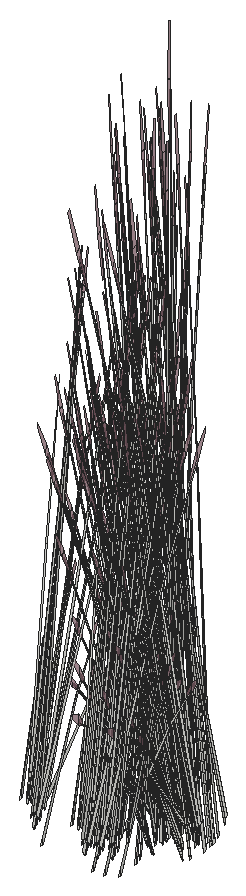
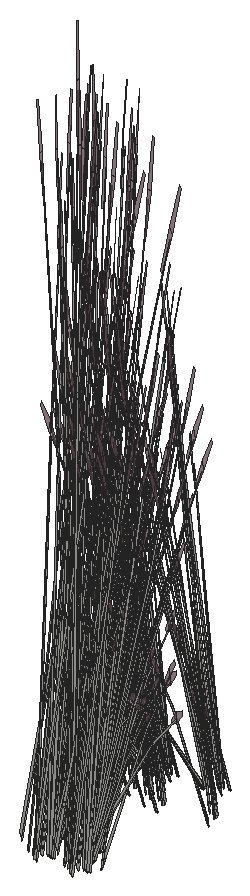
# SketchUp Ruby script. Lengths in inches.
U = 1.inch
M = Sketchup.active_model
def pt(a) = Geom::Point3d.new(a.map { |v| v * U })
def face(e, loops, mat)
  f = e.add_face(loops[0].map { |a| pt(a) })
  loops[1..].each { |l| e.add_face(l.map { |a| pt(a) }).erase! }
  f.material = f.back_material = mat if mat
  f
end
# faces: each face lists its corners as indices into pts; further lists are holes
def faces(e, pts, list, mat = nil) = list.each { |f| face(e, (f[0].is_a?(Array) ? f : [f]).map { |l| l.map { |i| pts[i] } }, mat) }
# xy, xz, yz: faces in a plane at the given z, y or x. An outline is a flat list of corners, or four numbers for a rectangle; further outlines are holes
def ring(l) = l.size == 4 ? [[l[0], l[1]], [l[2], l[1]], [l[2], l[3]], [l[0], l[3]]] : l.each_slice(2).to_a
def flat(e, list, mat, &to3) = list.each { |f| face(e, (f[0].is_a?(Array) ? f : [f]).map { |l| ring(l).map { |u, v| to3.(u, v) } }, mat) }
def xy(e, z, list, mat = nil) = flat(e, list, mat) { |x, y| [x, y, z] }
def xz(e, y, list, mat = nil) = flat(e, list, mat) { |x, z| [x, y, z] }
def yz(e, x, list, mat = nil) = flat(e, list, mat) { |y, z| [x, y, z] }
def lines(e, pts, list) = list.each { |a, b| e.add_line(pt(pts[a]), pt(pts[b])) }
# prism: a flat outline (further loops are holes) pulled along v
def prism(e, loops, v, mat = nil)
  f = face(e, loops, mat); d = Geom::Vector3d.new(v.map { |x| x * U })
  f.pushpull(f.normal.samedirection?(d) ? d.length : -d.length)
end
def box(e, o, s, mat = nil) = prism(e, [[o, [o[0] + s[0], o[1], o[2]], [o[0] + s[0], o[1] + s[1], o[2]], [o[0], o[1] + s[1], o[2]]]], [0, 0, s[2]], mat)
def at(x, y, z, deg = 0) = Geom::Transformation.translation(pt([x, y, z])) * Geom::Transformation.rotation(ORIGIN, Z_AXIS, deg.degrees)
def axes(o, x, y, z) = Geom::Transformation.new([*x, 0, *y, 0, *z, 0, *pt(o).to_a, 1])
def part(name) = M.definitions.add(name)
# library, detail: a bought-in or finely detailed component or shape, given as its bounding box
def library(name, o, s) = part(name).tap { |d| box(d.entities, o, s) }
def detail(e, o, s) = box(e.add_group.entities, o, s)
def put(e, d, t, mat = nil) = e.add_instance(d, t).tap { |i| i.material = mat if mat }
def group(e, t, mat = nil) = e.add_group.tap { |g| g.transformation = t; g.material = mat if mat }.entities
root = M.entities
M.materials.add("LightPink_Translucent").color = [144, 107, 117]
M.materials["LightPink_Translucent"].alpha = 0.75
c1 = part("blade")
p = [[2.15,0.21,22],[0,0.17,0],[0.09,0.45,0],[2.18,0.31,22],[2.29,0.31,22],[0.38,0.45,0],
  [2.48,0.24,33],[2.49,0.24,33],[2.48,0.22,33]]
faces(c1.entities,p,[[0,1,2,3],[4,5,2,3],[6,3,4,7],[8,0,3,6]])
c2 = part("seeds")
p = [[0.3,-0.1,1.38],[-0.01,-0.03,1.59],[-0.01,-0.03,0.03],[0.14,-0.07,-0.07],[0.29,-0.03,3],[0.15,0.01,3.11]]
faces(c2.entities,p,[[0,1,2,3],[1,0,4,5]],"LightPink_Translucent")
c3 = part("blade with seeds")
put(c3.entities,c1,at(0,0,0))
put(c3.entities,c2,axes([2.4,0.25,30.99],[1.5799,-0.05474,1.17369],[-0.12525,1.92788,0.29478],[-0.07173,-0.02425,1.56792]))
put(root,c3,axes([333.97,652.92,624.4375],[-0.00877,0.09229,1.74944],[0.24897,0.32105,-0.27667],[-0.06518,0.15182,0.14031]))
put(root,c3,axes([334.68,653.7,622.31],[0.11138,-0.07357,1.43002],[0.27499,0.22183,-0.30754],[-0.08185,0.19194,0.61141]))
put(root,c3,axes([334.79,652.99,624.25],[-0.23881,0.24554,-0.35414],[-0.22606,-0.28036,0.4572],[-0.0344,0.14245,0.87481]))
put(root,c3,axes([333.94,653.86,624.43],[0.04004,-0.02816,1.77383],[0.33095,0.18728,-0.16761],[-0.00778,0.15594,0.31391]))
put(root,c3,axes([334.95,652.73,625.0625],[-0.00918,0.43138,-0.7886],[-0.38672,-0.02897,0.09517],[-0.04081,0.18275,1.11556]))
put(root,c3,axes([334.95,653.94,622.49],[-0.00913,-0.2773,1.1486],[0.22824,0.19778,0.84392],[-0.04489,0.13217,0.25299]))
put(root,c3,axes([334.82,653.34,623.09],[0.00775,-0.24075,1.54345],[0.34877,0.12716,0.21329],[-0.03022,0.25658,0.72882]))
put(root,c3,axes([335.03,652.875,624.73],[0.25266,0.31335,-0.5672],[-0.2669,0.27442,-0.43934],[-0.03844,0.15921,1.08528]))
put(root,c3,axes([334.77,652.71,625.12],[0.3879,0.02311,-0.13498],[-0.0106,0.43749,-0.74919],[-0.02694,0.1685,1.13838]))
put(root,c3,axes([334.76,653.34,622.55],[0.32063,-0.08258,0.06507],[0.07371,0.33271,-0.86304],[-0.02033,0.16842,0.7736]))
put(root,c3,axes([335.32,652.42,623.6],[-0.00864,-0.17899,1.71376],[0.37441,0.11874,0.13857],[-0.02316,0.25508,0.73262]))
put(root,c3,axes([335.59,653.34,624.79],[-0.34777,-0.12192,0.53283],[0.11892,-0.40083,0.43934],[0.0209,0.15763,1.10256]))
put(root,c3,axes([339.11,661.4375,621.875],[0.14639,-0.01056,1.71376],[-0.09712,0.45778,0.13857],[-0.20862,-0.02831,0.73262]))
put(root,c3,axes([335.49,653.37,624.45],[-0.26007,0.1585,0.0643],[-0.12729,-0.28902,0.50621],[0.02512,0.1274,0.77189]))
put(root,c3,axes([335.55,653.28,621.22],[0.05712,-0.02538,1.76342],[0.34359,0.13968,-0.26939],[0.01005,0.15742,0.30037]))
put(root,c3,axes([335.625,653.42,624.25],[-0.1064,0.35863,-0.35414],[-0.31043,-0.1046,0.4572],[0.02846,0.14439,0.87481]))
put(root,c3,axes([335.4,654.06,624.4375],[0.04474,0.0751,1.74944],[0.36104,0.0295,-0.27667],[0.03631,0.16562,0.14031]))
put(root,c3,axes([339.55,661.01,622.98],[-0.35281,-0.01123,-0.71045],[0.0237,-0.47284,0.08574],[-0.14947,-0.0499,1.00501]))
put(root,c3,axes([339.26,661.125,620.59],[0.06891,0.12984,1.43002],[-0.15879,0.35293,-0.30754],[-0.16304,-0.08436,0.61141]))
put(root,c3,axes([339.39,660.7,621.875],[0.1311,0.08035,1.71376],[-0.27131,0.33708,0.13857],[-0.16909,-0.15206,0.73262]))
put(root,c3,axes([335.66,653.1,624.71],[0.16845,0.3792,-0.71045],[-0.34676,0.21133,0.08574],[0.03939,0.18322,1.00501]))
put(root,c3,axes([339.43,661.11,622.68],[-0.25628,0.30892,-0.51099],[-0.22444,-0.32634,-0.3958],[-0.13021,-0.047,0.97773]))
put(root,c3,axes([339.07,660.24,622.71],[0.02617,0.04654,1.77383],[-0.12614,0.41836,-0.16761],[-0.12775,0.00303,0.31391]))
put(root,c3,axes([335.78,653.18,624.4],[0.34695,0.11691,-0.51099],[-0.11892,0.40083,-0.3958],[0.03181,0.16138,0.97773]))
put(root,c3,axes([335.49,653.2,624.76],[0.34538,-0.21713,-0.1216],[0.16972,0.38536,-0.67495],[0.04557,0.16239,1.02557]))
put(root,c3,axes([339.36,659.96,622.72],[-0.07594,-0.00329,1.74944],[-0.24177,0.32918,-0.27667],[-0.129,-0.06726,0.14031]))
put(root,c3,axes([339.57,660.78,623.03],[-0.0189,0.47427,-0.1216],[-0.35781,-0.01296,-0.67495],[-0.13781,-0.03295,1.02557]))
put(root,c3,axes([339.34,660.82,622.53],[-0.20082,-0.29199,-0.35414],[0.2293,-0.2764,0.4572],[-0.1165,-0.04206,0.87481]))
put(root,c3,axes([338.85,661.52,620.77],[0.22533,-0.03337,1.1486],[-0.14293,0.29403,0.84392],[-0.11135,-0.04411,0.25299]))
put(root,c3,axes([338.43,652.92,623.9375],[-0.00877,0.09229,1.74944],[0.24897,0.32105,-0.27667],[-0.06518,0.15182,0.14031]))
put(root,c3,axes([339.31,660.71,623.09],[0.29147,-0.34417,0.53763],[0.25138,0.3655,0.4433],[-0.13675,-0.06349,1.11249]))
put(root,c3,axes([335.98,652.35,623.6],[-0.08068,-0.14973,1.71376],[0.3728,-0.12606,0.13857],[0.08426,0.23506,0.73262]))
put(root,c3,axes([339.4375,660.71,622.73],[0.01777,-0.35463,0.0643],[0.26836,0.00972,0.50621],[-0.1028,-0.03711,0.77189]))
put(root,c3,axes([340.2,662.66,620.06],[-0.36714,-0.07646,-0.62353],[0.07747,-0.47163,-0.16365],[-0.10956,-0.05715,1.37633]))
put(root,c3,axes([340.26,660.09,623.43],[-0.23555,0.44708,-0.13619],[-0.34112,-0.25757,-0.75594],[-0.11858,-0.12631,1.14864]))
put(root,c3,axes([339.62,660.97,623.05],[0.20082,0.29199,0.35414],[-0.2293,0.2764,-0.4572],[-0.1165,-0.04206,0.87481]))
put(root,c3,axes([340.16,660.45,622.98],[-0.30095,-0.22541,-0.71045],[0.21388,-0.395,0.08574],[-0.10904,-0.13459,1.00501]))
put(root,c3,axes([340.02,660.47,622.68],[-0.34827,0.11086,-0.51099],[-0.06092,-0.41983,-0.3958],[-0.09354,-0.12031,0.97773]))
put(root,c3,axes([339.14,653.7,621.81],[0.11138,-0.07357,1.43002],[0.27499,0.22183,-0.30754],[-0.08185,0.19194,0.61141]))
put(root,c3,axes([339.57,660.08,619.49],[-0.03419,0.06144,1.76342],[-0.3455,0.13246,-0.26939],[-0.08346,-0.12049,0.30037]))
put(root,c3,axes([339.26,652.99,623.75],[-0.23881,0.24554,-0.35414],[-0.22606,-0.28036,0.4572],[-0.0344,0.14245,0.87481]))
put(root,c3,axes([339.36,660.32,620.13],[-0.10181,0.3808,-0.03893],[-0.31336,-0.11714,-0.17649],[-0.04758,-0.06228,0.58215]))
put(root,c3,axes([340.17,659.03,622.71],[-0.00658,0.0559,1.77383],[-0.32474,0.20287,-0.16761],[-0.09556,-0.1037,0.31391]))
put(root,c3,axes([339.51,652.92,624.03],[-0.00877,0.09229,1.74944],[0.24897,0.32105,-0.27667],[-0.06518,0.15182,0.14031]))
put(root,c3,axes([338.4,653.86,623.93],[0.04004,-0.02816,1.77383],[0.33095,0.18728,-0.16761],[-0.00778,0.15594,0.31391]))
put(root,c3,axes([339.82,659.84,620.59],[-0.02137,0.15256,1.43002],[-0.31245,0.12771,-0.30754],[-0.07303,-0.19719,0.61141]))
put(root,c3,axes([339.93,660.24,621.875],[0.08068,0.14973,1.71376],[-0.3728,0.12606,0.13857],[-0.08426,-0.23506,0.73262]))
put(root,c3,axes([340.06,660.16,622.53],[-0.05451,-0.37564,-0.35414],[0.31161,-0.09919,0.4572],[-0.0837,-0.10765,0.87481]))
put(root,c3,axes([339.1875,662.06,620.375],[-0.44133,0,0],[0,-0.52122,-0.51607],[0,-0.11871,1.63711]))
put(root,c3,axes([339.41,652.73,624.5625],[-0.00918,0.43138,-0.7886],[-0.38672,-0.02897,0.09517],[-0.04081,0.18275,1.11556]))
put(root,c3,axes([339.41,653.94,621.99],[-0.00913,-0.2773,1.1486],[0.22824,0.19778,0.84392],[-0.04489,0.13217,0.25299]))
put(root,c3,axes([342.22,661.42,621.875],[0.14639,-0.01056,1.71376],[-0.09712,0.45778,0.13857],[-0.20862,-0.02831,0.73262]))
put(root,c3,axes([340.24,660.46,623.05],[0.05451,0.37564,0.35414],[-0.31161,0.09919,-0.4572],[-0.0837,-0.10765,0.87481]))
put(root,c3,axes([339.53,661.92,620.33],[-0.32829,0.39208,0.30756],[-0.32849,-0.38796,-0.36492],[-0.01146,-0.11134,1.64885]))
put(root,c3,axes([339.28,653.34,622.59],[0.00775,-0.24075,1.54345],[0.34877,0.12716,0.21329],[-0.03022,0.25658,0.72882]))
put(root,c3,axes([340.88,663,621.33],[0.305,0.18805,1.51261],[-0.29879,0.40513,0.59816],[-0.13384,-0.24012,1.26806]))
put(root,c3,axes([339.72,659.59,620.77],[0.18411,0.16231,1.1486],[-0.26813,0.09757,0.84392],[-0.05737,-0.12474,0.25299]))
put(root,c3,axes([340.39,662.51,620.21],[-0.21202,-0.39143,-0.44739],[0.32115,-0.27564,0.21531],[-0.06861,-0.04843,1.43643]))
put(root,c3,axes([340.22,653.7,621.91],[0.11138,-0.07357,1.43002],[0.27499,0.22183,-0.30754],[-0.08185,0.19194,0.61141]))
put(root,c3,axes([340.1,660.02,623.09],[0.39316,-0.11987,0.53763],[0.06823,0.47021,0.4433],[-0.09247,-0.13858,1.11249]))
put(root,c3,axes([339.49,652.875,624.23],[0.25266,0.31335,-0.5672],[-0.2669,0.27442,-0.43934],[-0.03844,0.15921,1.08528]))
put(root,c3,axes([340.19,660.12,622.73],[0.16041,-0.29625,0.0643],[0.22843,0.17248,0.50621],[-0.07385,-0.09498,0.77189]))
put(root,c3,axes([340.42,662.74,620.4375],[0.09355,-0.55261,-0.23429],[0.44354,0.09633,0.51271],[-0.0775,-0.07631,1.5644]))
put(root,c3,axes([339.23,652.71,624.62],[0.3879,0.02311,-0.13498],[-0.0106,0.43749,-0.74919],[-0.02694,0.1685,1.13838]))
put(root,c3,axes([340.33,652.99,623.84],[-0.23881,0.24554,-0.35414],[-0.22606,-0.28036,0.4572],[-0.0344,0.14245,0.87481]))
put(root,c3,axes([339.22,653.34,622.05],[0.32063,-0.08258,0.06507],[0.07371,0.33271,-0.86304],[-0.02033,0.16842,0.7736]))
put(root,c3,axes([340.54,659.24,622.72],[-0.05398,-0.06539,1.74944],[-0.36026,0.04145,-0.27667],[-0.0575,-0.15639,0.14031]))
put(root,c3,axes([339.29,661.7,620.02],[0,-0.46636,-0.49651],[0.39487,0,0],[0,-0.10622,1.57504]))
put(root,c3,axes([339.46,662.14,620.48],[0,0.46636,0.49651],[-0.39487,0,0],[0,-0.10622,1.57504]))
put(root,c3,axes([339.78,652.42,623.1],[-0.00864,-0.17899,1.71376],[0.37441,0.11874,0.13857],[-0.02316,0.25508,0.73262]))
put(root,c3,axes([342.66,660.99,622.98],[-0.35281,-0.01123,-0.71045],[0.0237,-0.47284,0.08574],[-0.14947,-0.0499,1.00501]))
put(root,c3,axes([339.48,653.86,624.03],[0.04004,-0.02816,1.77383],[0.33095,0.18728,-0.16761],[-0.00778,0.15594,0.31391]))
put(root,c3,axes([342.38,661.11,620.59],[0.06891,0.12984,1.43002],[-0.15879,0.35293,-0.30754],[-0.16304,-0.08436,0.61141]))
put(root,c3,axes([340.32,662.24,620.67],[-0.39748,-0.22252,-0.29095],[0.19139,-0.46966,-0.50002],[-0.01249,-0.11531,1.59708]))
put(root,c3,axes([342.5,660.68,621.875],[0.1311,0.08035,1.71376],[-0.27131,0.33708,0.13857],[-0.16909,-0.15206,0.73262]))
put(root,c3,axes([340.49,652.73,624.66],[-0.00918,0.43138,-0.7886],[-0.38672,-0.02897,0.09517],[-0.04081,0.18275,1.11556]))
put(root,c3,axes([340.84,652.92,624.42],[-0.00877,0.09229,1.74944],[0.24897,0.32105,-0.27667],[-0.06518,0.15182,0.14031]))
put(root,c3,axes([340.49,653.94,622.08],[-0.00913,-0.2773,1.1486],[0.22824,0.19778,0.84392],[-0.04489,0.13217,0.25299]))
put(root,c3,axes([340.14,661.77,620.1],[-0.14494,-0.47823,-0.69835],[0.41752,-0.17223,-0.18329],[-0.01602,-0.16194,1.54149]))
put(root,c3,axes([341.09,660.25,623.03],[-0.34538,0.21713,-0.1216],[-0.16972,-0.38536,-0.67495],[-0.04557,-0.16239,1.02557]))
put(root,c3,axes([340.79,660.27,622.68],[-0.34695,-0.11691,-0.51099],[0.11892,-0.40083,-0.3958],[-0.03181,-0.16138,0.97773]))
put(root,c3,axes([342.55,661.09,622.68],[-0.25628,0.30892,-0.51099],[-0.22444,-0.32634,-0.3958],[-0.13021,-0.047,0.97773]))
put(root,c3,axes([339.46,661.71,620.03],[0.24637,-0.29097,-0.30978],[0.24637,0.29097,0.30978],[0,-0.09372,1.38974]))
put(root,c3,axes([342.18,660.22,622.71],[0.02617,0.04654,1.77383],[-0.12614,0.41836,-0.16761],[-0.12775,0.00303,0.31391]))
put(root,c3,axes([340.57,659.83,620.13],[-0.2439,0.26754,-0.03893],[-0.22348,-0.29302,-0.17649],[-0.01573,-0.08303,0.58215]))
put(root,c3,axes([340.36,653.34,622.68],[0.00775,-0.24075,1.54345],[0.34877,0.12716,0.21329],[-0.03022,0.25658,0.72882]))
put(root,c3,axes([340.05,653.34,624.29],[-0.34777,-0.12192,0.53283],[0.11892,-0.40083,0.43934],[0.0209,0.15763,1.10256]))
put(root,c3,axes([342.48,659.94,622.72],[-0.07594,-0.00329,1.74944],[-0.24177,0.32918,-0.27667],[-0.129,-0.06726,0.14031]))
put(root,c3,axes([339.95,653.37,623.95],[-0.26007,0.1585,0.0643],[-0.12729,-0.28902,0.50621],[0.02512,0.1274,0.77189]))
put(root,c3,axes([340.36,662.37,620.72],[-0.17124,0.42022,0.44739],[-0.35581,-0.20224,-0.21531],[0,-0.09687,1.43643]))
put(root,c3,axes([340.92,660.35,622.98],[-0.16845,-0.3792,-0.71045],[0.34676,-0.21133,0.08574],[-0.03939,-0.18322,1.00501]))
put(root,c3,axes([342.68,660.76,623.03],[-0.0189,0.47427,-0.1216],[-0.35781,-0.01296,-0.67495],[-0.13781,-0.03295,1.02557]))
put(root,c3,axes([342.45,660.8,622.53],[-0.20082,-0.29199,-0.35414],[0.2293,-0.2764,0.4572],[-0.1165,-0.04206,0.87481]))
put(root,c3,axes([340.57,652.875,624.32],[0.25266,0.31335,-0.5672],[-0.2669,0.27442,-0.43934],[-0.03844,0.15921,1.08528]))
put(root,c3,axes([341.97,661.5,620.77],[0.22533,-0.03337,1.1486],[-0.14293,0.29403,0.84392],[-0.11135,-0.04411,0.25299]))
put(root,c3,axes([340.99,660.4,623.05],[-0.1064,0.35863,0.35414],[-0.31043,-0.1046,-0.4572],[-0.02846,-0.14439,0.87481]))
put(root,c3,axes([341.55,653.7,622.3],[0.11138,-0.07357,1.43002],[0.27499,0.22183,-0.30754],[-0.08185,0.19194,0.61141]))
put(root,c3,axes([340.01,653.28,620.72],[0.05712,-0.02538,1.76342],[0.34359,0.13968,-0.26939],[0.01005,0.15742,0.30037]))
put(root,c3,axes([340.31,652.71,624.71],[0.3879,0.02311,-0.13498],[-0.0106,0.43749,-0.74919],[-0.02694,0.1685,1.13838]))
put(root,c3,axes([340.08,653.42,623.75],[-0.1064,0.35863,-0.35414],[-0.31043,-0.1046,0.4572],[0.02846,0.14439,0.87481]))
put(root,c3,axes([340.3,653.34,622.14],[0.32063,-0.08258,0.06507],[0.07371,0.33271,-0.86304],[-0.02033,0.16842,0.7736]))
put(root,c3,axes([342.42,660.6875,623.09],[0.29147,-0.34417,0.53763],[0.25138,0.3655,0.4433],[-0.13675,-0.06349,1.11249]))
put(root,c3,axes([340.86,652.42,623.19],[-0.00864,-0.17899,1.71376],[0.37441,0.11874,0.13857],[-0.02316,0.25508,0.73262]))
put(root,c3,axes([340.63,659.51,619.49],[-0.0592,0.0168,1.76342],[-0.32738,-0.18913,-0.26939],[0.00549,-0.15776,0.30037]))
put(root,c3,axes([341.67,652.99,624.23],[-0.23881,0.24554,-0.35414],[-0.22606,-0.28036,0.4572],[-0.0344,0.14245,0.87481]))
put(root,c3,axes([340.95,660.02,622.53],[0.1064,-0.35863,-0.35414],[0.31043,0.1046,0.4572],[-0.02846,-0.14439,0.87481]))
put(root,c3,axes([340.43,661.96,620.36],[0.15345,0.52148,0.45755],[-0.43845,0.18134,0.17955],[0.00536,-0.09582,1.58856]))
put(root,c3,axes([339.86,654.06,623.9375],[0.04474,0.0751,1.74944],[0.36104,0.0295,-0.27667],[0.03631,0.16562,0.14031]))
put(root,c3,axes([340.36,661.89,620.21],[0.17124,-0.42022,-0.44739],[0.35581,0.20224,0.21531],[0,-0.09687,1.43643]))
put(root,c3,axes([342.55,660.68,622.73],[0.01777,-0.35463,0.0643],[0.26836,0.00972,0.50621],[-0.1028,-0.03711,0.77189]))
put(root,c3,axes([340.82,653.86,624.42],[0.04004,-0.02816,1.77383],[0.33095,0.18728,-0.16761],[-0.00778,0.15594,0.31391]))
put(root,c3,axes([343.3125,662.64,620.06],[-0.36714,-0.07646,-0.62353],[0.07747,-0.47163,-0.16365],[-0.10956,-0.05715,1.37633]))
put(root,c3,axes([343.38,660.07,623.43],[-0.23555,0.44708,-0.13619],[-0.34112,-0.25757,-0.75594],[-0.11858,-0.12631,1.14864]))
put(root,c3,axes([342.74,660.95,623.05],[0.20082,0.29199,0.35414],[-0.2293,0.2764,-0.4572],[-0.1165,-0.04206,0.87481]))
put(root,c3,axes([343.28,660.43,622.98],[-0.30095,-0.22541,-0.71045],[0.21388,-0.395,0.08574],[-0.10904,-0.13459,1.00501]))
put(root,c3,axes([343.14,660.44,622.68],[-0.34827,0.11086,-0.51099],[-0.06092,-0.41983,-0.3958],[-0.09354,-0.12031,0.97773]))
put(root,c3,axes([341.83,652.73,625.05],[-0.00918,0.43138,-0.7886],[-0.38672,-0.02897,0.09517],[-0.04081,0.18275,1.11556]))
put(root,c3,axes([340.12,653.1,624.21],[0.16845,0.3792,-0.71045],[-0.34676,0.21133,0.08574],[0.03939,0.18322,1.00501]))
put(root,c3,axes([341.125,653.34,624.38],[-0.34777,-0.12192,0.53283],[0.11892,-0.40083,0.43934],[0.0209,0.15763,1.10256]))
put(root,c3,axes([341.08,660.08,622.73],[0.26007,-0.1585,0.0643],[0.12729,0.28902,0.50621],[-0.02512,-0.1274,0.77189]))
put(root,c3,axes([341.82,653.94,622.47],[-0.00913,-0.2773,1.1486],[0.22824,0.19778,0.84392],[-0.04489,0.13217,0.25299]))
put(root,c3,axes([342.6875,660.0625,619.49],[-0.03419,0.06144,1.76342],[-0.3455,0.13246,-0.26939],[-0.08346,-0.12049,0.30037]))
put(root,c3,axes([340.98,662.01,620.21],[0,-0.53961,0],[0.44133,0,0],[0,0,1.79456]))
put(root,c3,axes([341.03,653.37,624.05],[-0.26007,0.1585,0.0643],[-0.12729,-0.28902,0.50621],[0.02512,0.1274,0.77189]))
put(root,c3,axes([340.99,660.11,622.73],[0.34777,0.12192,0.48003],[-0.11892,0.40083,0.3958],[-0.0209,-0.15763,0.9933]))
put(root,c3,axes([340.57,662.1,620.43],[0.39767,0.22603,0.24065],[-0.19139,0.46966,0.50002],[0,-0.10827,1.60543]))
put(root,c3,axes([340.45,661.79,620.72],[-0.38326,0.02879,0.44739],[-0.03466,-0.47788,-0.21531],[0.06861,-0.04843,1.43643]))
put(root,c3,axes([341.7,653.34,623.07],[0.00775,-0.24075,1.54345],[0.34877,0.12716,0.21329],[-0.03022,0.25658,0.72882]))
put(root,c3,axes([340.24,653.18,623.9],[0.34695,0.11691,-0.51099],[-0.11892,0.40083,-0.3958],[0.03181,0.16138,0.97773]))
put(root,c3,axes([339.95,653.2,624.26],[0.34538,-0.21713,-0.1216],[0.16972,0.38536,-0.67495],[0.04557,0.16239,1.02557]))
put(root,c3,axes([340.08,660.4,620.375],[-0.22066,-0.46731,0],[0.36918,-0.26061,-0.51607],[0.08408,-0.05936,1.63711]))
put(root,c3,axes([342.47,660.3,620.13],[-0.10181,0.3808,-0.03893],[-0.31336,-0.11714,-0.17649],[-0.04758,-0.06228,0.58215]))
put(root,c3,axes([341.09,653.28,620.81],[0.05712,-0.02538,1.76342],[0.34359,0.13968,-0.26939],[0.01005,0.15742,0.30037]))
put(root,c3,axes([341.16,653.42,623.84],[-0.1064,0.35863,-0.35414],[-0.31043,-0.1046,0.4572],[0.02846,0.14439,0.87481]))
put(root,c3,axes([343.29,659.01,622.71],[-0.00658,0.0559,1.77383],[-0.32474,0.20287,-0.16761],[-0.09556,-0.1037,0.31391]))
put(root,c3,axes([341.01,659.27,620.77],[0.04528,0.27194,1.1486],[-0.25117,-0.15062,0.84392],[0.02703,-0.13924,0.25299]))
put(root,c3,axes([341.91,652.875,624.71],[0.25266,0.31335,-0.5672],[-0.2669,0.27442,-0.43934],[-0.03844,0.15921,1.08528]))
put(root,c3,axes([342.9375,659.82,620.59],[-0.02137,0.15256,1.43002],[-0.31245,0.12771,-0.30754],[-0.07303,-0.19719,0.61141]))
put(root,c3,axes([343.04,660.21,621.875],[0.08068,0.14973,1.71376],[-0.3728,0.12606,0.13857],[-0.08426,-0.23506,0.73262]))
put(root,c3,axes([340.78,661.67,620.36],[-0.29264,0.42323,0.45755],[-0.34767,-0.3736,0.17955],[0.07055,-0.04224,1.58856]))
put(root,c3,axes([342.78,652.92,624.44],[-0.00877,0.09229,1.74944],[0.24897,0.32105,-0.27667],[-0.06518,0.15182,0.14031]))
put(root,c3,axes([343.17,660.14,622.53],[-0.05451,-0.37564,-0.35414],[0.31161,-0.09919,0.4572],[-0.0837,-0.10765,0.87481]))
put(root,c3,axes([342.3,662.04,620.375],[-0.44133,0,0],[0,-0.52122,-0.51607],[0,-0.11871,1.63711]))
put(root,c3,axes([341.64,652.71,625.1],[0.3879,0.02311,-0.13498],[-0.0106,0.43749,-0.74919],[-0.02694,0.1685,1.13838]))
put(root,c3,axes([342.08,659.71,622.71],[-0.03584,0.03562,1.77383],[-0.35118,-0.12018,-0.16761],[-0.01271,-0.15545,0.31391]))
put(root,c3,axes([340.94,654.06,624.03],[0.04474,0.0751,1.74944],[0.36104,0.0295,-0.27667],[0.03631,0.16562,0.14031]))
put(root,c3,axes([341.81,660.74,623.03],[-0.3879,-0.02311,-0.1216],[0.0106,-0.43749,-0.67495],[0.02694,-0.1685,1.02557]))
put(root,c3,axes([341.63,653.34,622.53],[0.32063,-0.08258,0.06507],[0.07371,0.33271,-0.86304],[-0.02033,0.16842,0.7736]))
put(root,c3,axes([342.19,652.42,623.58],[-0.00864,-0.17899,1.71376],[0.37441,0.11874,0.13857],[-0.02316,0.25508,0.73262]))
put(root,c3,axes([343.36,660.44,623.05],[0.05451,0.37564,0.35414],[-0.31161,0.09919,-0.4572],[-0.0837,-0.10765,0.87481]))
put(root,c3,axes([341.66,660.81,623.05],[-0.23881,0.24554,0.35414],[-0.22606,-0.28036,-0.4572],[0.0344,-0.14245,0.87481]))
put(root,c3,axes([342.64,661.9,620.33],[-0.32829,0.39208,0.30756],[-0.32849,-0.38796,-0.36492],[-0.01146,-0.11134,1.64885]))
put(root,c3,axes([340.52,661.6875,620.67],[-0.04113,-0.53214,-0.29095],[0.42835,-0.03218,-0.50002],[0.07543,-0.07088,1.59708]))
put(root,c3,axes([340.4375,652.35,623.1],[-0.08068,-0.14973,1.71376],[0.3728,-0.12606,0.13857],[0.08426,0.23506,0.73262]))
put(root,c3,axes([341.54,660.57,622.68],[-0.25266,-0.31335,-0.51099],[0.2669,-0.27442,-0.3958],[0.03844,-0.15921,0.97773]))
put(root,c3,axes([344,662.98,621.33],[0.305,0.18805,1.51261],[-0.29879,0.40513,0.59816],[-0.13384,-0.24012,1.26806]))
put(root,c3,axes([342.83,659.57,620.77],[0.18411,0.16231,1.1486],[-0.26813,0.09757,0.84392],[-0.05737,-0.12474,0.25299]))
put(root,c3,axes([343.5,662.49,620.21],[-0.21202,-0.39143,-0.44739],[0.32115,-0.27564,0.21531],[-0.06861,-0.04843,1.43643]))
put(root,c3,axes([341.19,653.1,624.3],[0.16845,0.3792,-0.71045],[-0.34676,0.21133,0.08574],[0.03939,0.18322,1.00501]))
put(root,c3,axes([340.46,660.51,620.03],[0.32928,0.11539,-0.30978],[-0.08291,0.40636,0.30978],[0.06638,-0.04686,1.38974]))
put(root,c3,axes([343.22,660,623.09],[0.39316,-0.11987,0.53763],[0.06823,0.47021,0.4433],[-0.09247,-0.13858,1.11249]))
put(root,c3,axes([341.38,660.02,620.59],[-0.10032,0.0944,1.43002],[-0.30046,-0.16522,-0.30754],[0.05569,-0.20547,0.61141]))
put(root,c3,axes([343.49,653.7,622.32],[0.11138,-0.07357,1.43002],[0.27499,0.22183,-0.30754],[-0.08185,0.19194,0.61141]))
put(root,c3,axes([343.31,660.1,622.73],[0.16041,-0.29625,0.0643],[0.22843,0.17248,0.50621],[-0.07385,-0.09498,0.77189]))
put(root,c3,axes([340.38,660.32,620.02],[0.33032,-0.23318,-0.49651],[0.19744,0.41812,0],[0.07523,-0.05311,1.57504]))
put(root,c3,axes([343.53,662.72,620.4375],[0.09355,-0.55261,-0.23429],[0.44354,0.09633,0.51271],[-0.0775,-0.07631,1.5644]))
put(root,c3,axes([342.46,653.34,624.77],[-0.34777,-0.12192,0.53283],[0.11892,-0.40083,0.43934],[0.0209,0.15763,1.10256]))
put(root,c3,axes([341.32,653.18,624],[0.34695,0.11691,-0.51099],[-0.11892,0.40083,-0.3958],[0.03181,0.16138,0.97773]))
put(root,c3,axes([341.02,653.2,624.35],[0.34538,-0.21713,-0.1216],[0.16972,0.38536,-0.67495],[0.04557,0.16239,1.02557]))
put(root,c3,axes([342.37,653.37,624.4375],[-0.26007,0.1585,0.0643],[-0.12729,-0.28902,0.50621],[0.02512,0.1274,0.77189]))
put(root,c3,axes([341.52,660.76,620.48],[-0.33032,-0.23318,0.49651],[0.19744,-0.41812,0],[0.07523,0.05311,1.57504]))
put(root,c3,axes([341.62,660.72,622.98],[0.00918,-0.43138,-0.71045],[0.38672,0.02897,0.08574],[0.04081,-0.18275,1.00501]))
put(root,c3,axes([343.66,659.22,622.72],[-0.05398,-0.06539,1.74944],[-0.36026,0.04145,-0.27667],[-0.0575,-0.15639,0.14031]))
put(root,c3,axes([342.4,661.68,620.02],[0,-0.46636,-0.49651],[0.39487,0,0],[0,-0.10622,1.57504]))
put(root,c3,axes([342.57,662.12,620.48],[0,0.46636,0.49651],[-0.39487,0,0],[0,-0.10622,1.57504]))
put(root,c3,axes([343.6,652.99,624.25],[-0.23881,0.24554,-0.35414],[-0.22606,-0.28036,0.4572],[-0.0344,0.14245,0.87481]))
put(root,c3,axes([343.43,662.22,620.67],[-0.39748,-0.22252,-0.29095],[0.19139,-0.46966,-0.50002],[-0.01249,-0.11531,1.59708]))
put(root,c3,axes([342.75,653.86,624.43],[0.04004,-0.02816,1.77383],[0.33095,0.18728,-0.16761],[-0.00778,0.15594,0.31391]))
put(root,c3,axes([342.42,653.28,621.2],[0.05712,-0.02538,1.76342],[0.34359,0.13968,-0.26939],[0.01005,0.15742,0.30037]))
put(root,c3,axes([342.5,653.42,624.23],[-0.1064,0.35863,-0.35414],[-0.31043,-0.1046,0.4572],[0.02846,0.14439,0.87481]))
put(root,c3,axes([341.78,660.46,622.53],[0.23881,-0.24554,-0.35414],[0.22606,0.28036,0.4572],[0.0344,-0.14245,0.87481]))
put(root,c3,axes([341.87,660.58,622.73],[0.29004,0.02173,0.0643],[-0.00795,0.32812,0.50621],[0.03035,-0.12569,0.77189]))
put(root,c3,axes([343.26,661.75,620.1],[-0.14494,-0.47823,-0.69835],[0.41752,-0.17223,-0.18329],[-0.01602,-0.16194,1.54149]))
put(root,c3,axes([344.21,660.23,623.03],[-0.34538,0.21713,-0.1216],[-0.16972,-0.38536,-0.67495],[-0.04557,-0.16239,1.02557]))
put(root,c3,axes([343.91,660.25,622.68],[-0.34695,-0.11691,-0.51099],[0.11892,-0.40083,-0.3958],[-0.03181,-0.16138,0.97773]))
put(root,c3,axes([342.16,660.04,622.72],[-0.00341,-0.09282,1.74944],[-0.28775,-0.26825,-0.27667],[0.04449,-0.16261,0.14031]))
put(root,c3,axes([340.78,661.28,620.06],[0.23773,-0.35053,-0.62353],[0.29532,0.31785,-0.16365],[0.09526,-0.08744,1.37633]))
put(root,c3,axes([341.78,660.55,622.73],[0.25132,0.3182,0.48003],[-0.2669,0.27442,0.3958],[0.04636,-0.14929,0.9933]))
put(root,c3,axes([343.76,652.73,625.0625],[-0.00918,0.43138,-0.7886],[-0.38672,-0.02897,0.09517],[-0.04081,0.18275,1.11556]))
put(root,c3,axes([343.75,653.94,622.49],[-0.00913,-0.2773,1.1486],[0.22824,0.19778,0.84392],[-0.04489,0.13217,0.25299]))
put(root,c3,axes([342.57,661.69,620.03],[0.24637,-0.29097,-0.30978],[0.24637,0.29097,0.30978],[0,-0.09372,1.38974]))
put(root,c3,axes([343.68,659.8125,620.13],[-0.2439,0.26754,-0.03893],[-0.22348,-0.29302,-0.17649],[-0.01573,-0.08303,0.58215]))
put(root,c3,axes([341.52,652.35,623.19],[-0.08068,-0.14973,1.71376],[0.3728,-0.12606,0.13857],[0.08426,0.23506,0.73262]))
put(root,c3,axes([342.28,654.06,624.42],[0.04474,0.0751,1.74944],[0.36104,0.0295,-0.27667],[0.03631,0.16562,0.14031]))
put(root,c3,axes([343.47,662.35,620.72],[-0.17124,0.42022,0.44739],[-0.35581,-0.20224,-0.21531],[0,-0.09687,1.43643]))
